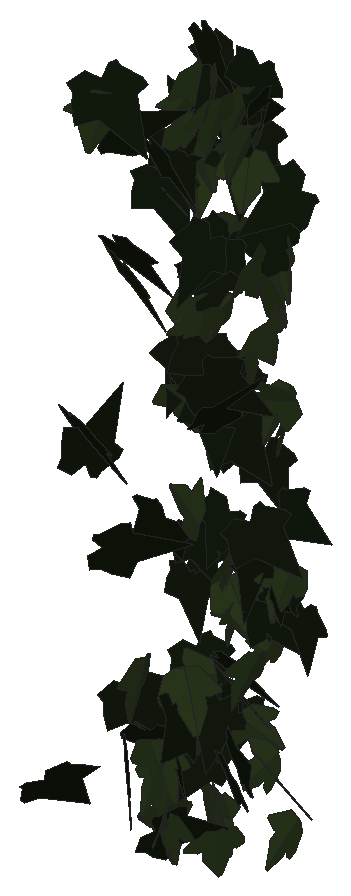
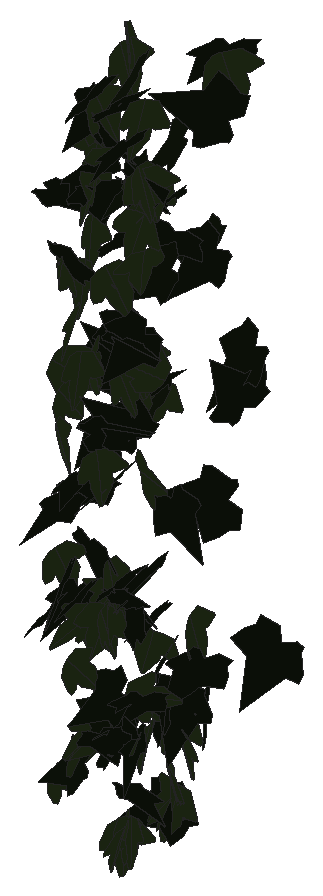
# SketchUp Ruby script. Lengths in inches.
U = 1.inch
M = Sketchup.active_model
def pt(a) = Geom::Point3d.new(a.map { |v| v * U })
def face(e, loops, mat)
  f = e.add_face(loops[0].map { |a| pt(a) })
  loops[1..].each { |l| e.add_face(l.map { |a| pt(a) }).erase! }
  f.material = f.back_material = mat if mat
  f
end
# faces: each face lists its corners as indices into pts; further lists are holes
def faces(e, pts, list, mat = nil) = list.each { |f| face(e, (f[0].is_a?(Array) ? f : [f]).map { |l| l.map { |i| pts[i] } }, mat) }
# xy, xz, yz: faces in a plane at the given z, y or x. An outline is a flat list of corners, or four numbers for a rectangle; further outlines are holes
def ring(l) = l.size == 4 ? [[l[0], l[1]], [l[2], l[1]], [l[2], l[3]], [l[0], l[3]]] : l.each_slice(2).to_a
def flat(e, list, mat, &to3) = list.each { |f| face(e, (f[0].is_a?(Array) ? f : [f]).map { |l| ring(l).map { |u, v| to3.(u, v) } }, mat) }
def xy(e, z, list, mat = nil) = flat(e, list, mat) { |x, y| [x, y, z] }
def xz(e, y, list, mat = nil) = flat(e, list, mat) { |x, z| [x, y, z] }
def yz(e, x, list, mat = nil) = flat(e, list, mat) { |y, z| [x, y, z] }
def lines(e, pts, list) = list.each { |a, b| e.add_line(pt(pts[a]), pt(pts[b])) }
# prism: a flat outline (further loops are holes) pulled along v
def prism(e, loops, v, mat = nil)
  f = face(e, loops, mat); d = Geom::Vector3d.new(v.map { |x| x * U })
  f.pushpull(f.normal.samedirection?(d) ? d.length : -d.length)
end
def box(e, o, s, mat = nil) = prism(e, [[o, [o[0] + s[0], o[1], o[2]], [o[0] + s[0], o[1] + s[1], o[2]], [o[0], o[1] + s[1], o[2]]]], [0, 0, s[2]], mat)
def at(x, y, z, deg = 0) = Geom::Transformation.translation(pt([x, y, z])) * Geom::Transformation.rotation(ORIGIN, Z_AXIS, deg.degrees)
def axes(o, x, y, z) = Geom::Transformation.new([*x, 0, *y, 0, *z, 0, *pt(o).to_a, 1])
def part(name) = M.definitions.add(name)
# library, detail: a bought-in or finely detailed component or shape, given as its bounding box
def library(name, o, s) = part(name).tap { |d| box(d.entities, o, s) }
def detail(e, o, s) = box(e.add_group.entities, o, s)
def put(e, d, t, mat = nil) = e.add_instance(d, t).tap { |i| i.material = mat if mat }
def group(e, t, mat = nil) = e.add_group.tap { |g| g.transformation = t; g.material = mat if mat }.entities
root = M.entities
M.materials.add("efeu1").color = [18, 25, 13]
M.materials.add("efeu2").color = [43, 57, 29]
c1 = part("ivyleaf_9")
p = [[1.54,2.16,1.25],[1.36,2.04,1.19],[-0.21,0.99,0.68],[-0.71,1.11,0.82],[-0.85,0.86,0.67],[-0.8,0.17,0.21],
  [-0.9,-0.01,0.1],[-0.67,-0.16,-0.02],[-0.08,-0.08,-0.05],[-0.03,-0.6,-0.4],[0.65,-0.88,-0.66],[0.83,-0.6,-0.49],
  [1.29,-0.42,-0.43],[1.8125,-0.07,-0.26],[1.21,0.44,0.15]]
faces(c1.entities,p,[[0,1,2,3,4,5,6,7,8,9,10,11,12,13,14]],"efeu1")
c2 = part("ivyleaf_10")
p = [[0,0.5,-0.03],[-0.0625,2.02,-0.43],[-0.19,2.01,-0.46],[-0.54,1.05,-0.29],[-0.52,0.625,-0.18],[-0.83,0.76,-0.28],
  [-1.16,0.64,-0.33],[-1.15,0.33,-0.24],[-0.77,-0.39,0.02],[-0.3,-0.51,0.16],[0.04,-0.48,0.23],[-0.02,2.01,-0.4375],
  [-0.06,2.01,-0.43],[0.04,-0.49,0.23],[0.67,-0.49,0.14],[1.38,0.36,-0.2],[1.375,0.51,-0.24],[0.81,0.65,-0.19],
  [0.62,0.59,-0.15],[0.6,1.09,-0.28],[0.5,1.23,-0.31]]
faces(c2.entities,p,[[0,1,2,3,4,5,6,7,8,9,10],[11,12,0,13,14,15,16,17,18,19,20]],"efeu2")
put(root,c1,axes([509.43,133.33,219.33],[-0.07106,-0.77175,0.46903],[0.10896,-0.47437,-0.76402],[0.8965,-0.00352,0.13004]))
put(root,c2,axes([510.06,132.71,207.74],[-0.8093,0.2525,0.27731],[-0.29187,0.03106,-0.82047],[-0.26852,-0.79478,0.05603]))
put(root,c1,axes([509.6,125.68,225.125],[-0.26044,-0.40713,1.01858],[0.82552,0.62963,0.46794],[-0.79417,0.788,0.15237]))
put(root,c2,axes([509.68,132.23,235],[0.34261,0.90145,-0.01403],[-0.024,-0.00589,-0.96415],[-0.90124,0.34285,0.02034]))
put(root,c1,axes([510.07,132.63,209.49],[-0.87413,-0.23226,-0.09111],[0.08835,0.03251,-0.87568],[0.25312,-0.81346,-0.00898]))
put(root,c1,axes([509.39,133.1,217.37],[-0.07665,0.02325,0.83497],[0.35529,-0.73444,0.05236],[0.79136,0.33199,0.05737]))
put(root,c1,axes([509.72,123.07,212.36],[0.6654,0.8894,0.22266],[0.13803,0.17192,-1.12521],[-0.97831,0.62918,-0.00731]))
put(root,c1,axes([509.26,131.03,234.0625],[0.93232,-0.34092,0.09087],[0.07451,-0.06071,-0.9922],[0.34487,0.93477,-0.0313]))
put(root,c2,axes([510.03,131.67,238.36],[-0.56572,-0.76176,0.26306],[-0.04096,-0.29381,-0.93889],[0.80486,-0.55038,0.13712]))
put(root,c1,axes([509.43,127.84,233.51],[1.09135,0.08087,-0.04492],[-0.04662,-0.00205,-1.05429],[-0.08735,1.01143,0.00146]))
put(root,c1,axes([510.04,132.28,212.05],[0.60792,0.03971,-0.70162],[-0.70045,0.1091,-0.60073],[0.0567,0.92192,0.10131]))
put(root,c1,axes([509.56,128.4,213.99],[-0.05655,-0.48604,-0.89596],[0.09111,0.85737,-0.50839],[1.06439,-0.09921,-0.00408]))
put(root,c1,axes([509.5,130.4,235.42],[-0.36524,-0.489,-0.76479],[0.59667,0.49718,-0.60806],[0.74408,-0.63872,0.1122]))
put(root,c2,axes([510.03,131.84,238.53],[0.0869,-0.97179,0.05974],[-0.00173,-0.06013,-0.97565],[0.97363,0.08663,-0.00707]))
put(root,c2,axes([509.9375,131.73,211.81],[-0.2319,0.86942,0.06748],[-0.10839,0.04173,-0.92693],[-0.93532,-0.2204,0.09069]))
put(root,c2,axes([510.45,131.67,213.4],[-0.11436,-0.10303,0.92284],[-0.44905,-0.80772,-0.14582],[0.81277,-0.46076,0.04928]))
put(root,c1,axes([510.33,133.125,218.96],[-0.86955,-0.17617,-0.02814],[0.03969,-0.04159,-0.85568],[0.18836,-0.80452,0.0504]))
put(root,c2,axes([510.09,129.67,207.88],[-1.06171,0.04755,-0.05074],[0.05296,0.0039,-1.02356],[-0.05108,-0.98427,-0.0065]))
put(root,c1,axes([509.62,132.41,213.9375],[0.01797,-0.70626,-0.60136],[0.21065,0.58886,-0.68529],[0.90336,-0.12327,0.17176]))
put(root,c1,axes([510.6875,130.98,237.37],[0.05271,0.33885,0.90179],[-0.69809,0.63722,-0.22114],[-0.72358,-0.59008,0.27904]))
put(root,c1,axes([509.74,131.83,217.45],[0.14195,-0.88574,-0.02827],[-0.00305,0.02814,-0.89704],[0.88618,0.14198,0.00144]))
put(root,c1,axes([510.6875,129,221.5],[0.2465,0.28682,-0.9281],[-0.88422,-0.38625,-0.34688],[-0.49296,0.83623,0.15811]))
put(root,c2,axes([510.39,129.7,207.65],[0.01164,-0.02182,1.01459],[-0.47332,0.89742,0.02473],[-0.89769,-0.47347,0.00012]))
put(root,c2,axes([510.15,131.92,236.31],[-0.9515,0.00766,-0.18123],[0.17924,-0.10887,-0.94566],[-0.02784,-0.96247,0.10552]))
put(root,c1,axes([509.93,131.95,231.05],[0.75543,0.52185,0.13154],[0.12521,0.05604,-0.90725],[-0.56624,0.70861,-0.02512]))
put(root,c2,axes([510.16,129.66,208.82],[0.74121,-0.70278,0.04986],[0.04945,-0.02228,-1.02144],[0.75916,0.68762,0.01785]))
put(root,c2,axes([509.8,131.42,228.96],[-0.2816,-0.37519,0.82169],[0.43763,0.67881,0.47432],[-0.83712,0.48108,-0.02844]))
put(root,c1,axes([509.84,124.74,227.29],[1.17306,-0.10964,-0.31105],[-0.31406,0.09259,-1.1336],[0.14045,1.12278,0.06311]))
put(root,c1,axes([509.82,130.72,236.91],[0.20947,-0.8926,-0.17498],[0.03574,0.17887,-0.94723],[0.98033,0.1842,0.07192]))
put(root,c2,axes([510.24,128.96,210.45],[0.8597,-0.59571,-0.01232],[-0.00625,0.01204,-1.03399],[0.64346,0.79601,0.00642]))
put(root,c2,axes([510.55,125.64,241.05],[-0.5616,-0.88248,0.33406],[-0.10765,-0.31323,-1.06278],[1.00852,-0.52485,0.07258]))
put(root,c1,axes([509.96,131.55,219.66],[0.36728,-0.74157,-0.37263],[-0.08365,0.37233,-0.82343],[0.8257,0.36758,0.08232]))
put(root,c1,axes([510.36,128.68,212.2],[0.83054,0.53659,-0.41955],[-0.36622,-0.21894,-0.97513],[-0.62574,0.84035,0.01384]))
put(root,c2,axes([510.28,128.0625,215.23],[0.20983,-0.98068,0.28092],[0.19545,-0.23728,-1.03132],[1.08105,0.23325,0.13194]))
put(root,c1,axes([510.21,133.48,219.61],[-0.22952,-0.81169,0.32932],[0.02334,-0.34598,-0.83649],[0.87564,-0.20353,0.10862]))
put(root,c1,axes([509.86,127.74,211.46],[-0.0249,-0.0004,-1.09458],[1.07455,-0.34331,-0.02253],[-0.37067,-0.99519,0.00821]))
put(root,c1,axes([509.76,126.68,220.91],[0.30691,0.57861,-0.88494],[0.33021,0.79541,0.66871],[1.06112,-0.41488,0.04786]))
put(root,c1,axes([510.07,129.45,207.47],[0.03422,0.43216,-0.90682],[0.07695,0.86903,0.45064],[1.0482,-0.07791,-0.00347]))
put(root,c1,axes([510.42,132.61,230.91],[-0.71795,-0.46742,-0.41007],[0.43629,0.06763,-0.84093],[0.44305,-0.82404,0.16358]))
put(root,c2,axes([510.62,132.46,229.02],[-0.01852,-0.91326,0.22885],[-0.0026,-0.22884,-0.91344],[0.94149,-0.0186,0.00198]))
put(root,c2,axes([510.41,128.92,211.3],[-1.0325,-0.04654,-0.30942],[0.32515,-0.16941,-0.97855],[-0.00712,-0.98681,0.18259]))
put(root,c2,axes([510.4,130.76,237.77],[-0.51607,-0.69102,-0.53281],[0.39573,0.36636,-0.85844],[0.77769,-0.64498,0.08324]))
put(root,c2,axes([510.07,132.96,207.2],[0.16278,-0.33966,0.83601],[0.78088,-0.37271,-0.30347],[0.45222,0.76583,0.22309]))
put(root,c2,axes([510.58,132.67,207.12],[-0.21816,0.84236,0.01689],[-0.00053,0.01659,-0.90088],[-0.90992,-0.20198,-0.00353]))
put(root,c1,axes([509.91,126.51,239.08],[0.32091,-0.01017,1.09752],[1.10805,0.25969,-0.29783],[-0.26708,1.06514,0.08309]))
put(root,c1,axes([510.58,130.75,227.85],[-0.32285,-0.85758,0.21738],[0.00785,-0.23416,-0.91216],[0.88466,-0.31089,0.08742]))
put(root,c2,axes([510.77,131.05,227.35],[0.18598,-0.8146,-0.43777],[0.11773,0.46376,-0.81294],[0.91725,0.10564,0.19311]))
put(root,c2,axes([510.9375,130.98,229.44],[-0.33356,-0.93089,0.08302],[-0.02373,-0.07969,-0.98883],[0.93428,-0.33438,0.00452]))
put(root,c1,axes([510.31,130.76,226.78],[0.44544,-0.77207,0.27374],[0.1962,-0.20197,-0.8889],[0.79532,0.48224,0.06597]))
put(root,c1,axes([510.26,132.15,226.25],[-0.01284,-0.03101,0.9233],[0.9576,-0.05476,0.01036],[0.05873,0.88618,0.03295]))
put(root,c1,axes([510.17,127.29,232.98],[0.63011,-0.72767,0.43253],[0.32063,-0.29446,-0.96895],[0.8465,0.6532,0.04505]))
put(root,c1,axes([510.74,132.4375,212.54],[-0.6482,-0.15584,-0.66212],[0.64227,0.16097,-0.66665],[0.224,-0.91249,-0.00452]))
put(root,c1,axes([510.47,125.59,241.98],[0.09469,-0.8526,-0.6817],[0.26966,0.65582,-0.85243],[1.12974,-0.08508,0.2606]))
put(root,c2,axes([511.23,131.59,206.63],[-0.54604,-0.76578,-0.05381],[0.0381,0.03892,-0.94048],[0.76672,-0.54731,0.00841]))
put(root,c2,axes([511.12,129.49,226.93],[-0.84642,-0.34341,-0.21699],[0.20364,0.07523,-0.9134],[0.35149,-0.87054,0.00667]))
put(root,c1,axes([510.83,131.1,238.03],[0.83199,-0.46646,-0.20758],[-0.17598,0.11057,-0.95378],[0.47928,0.85034,0.01014]))
put(root,c1,axes([511.9375,132.75,225.93],[-0.50923,-0.44858,-0.64625],[-0.41032,-0.50536,0.67411],[-0.67119,0.64928,0.0782]))
put(root,c2,axes([511.23,130.31,240.6],[-0.31499,-0.91313,-0.34822],[0.22971,0.28643,-0.9589],[0.9499,-0.37207,0.11642]))
put(root,c2,axes([511.6,132.06,233.33],[-0.52405,-0.70315,0.39512],[-0.23706,-0.31611,-0.87695],[0.77094,-0.57517,-0.00108]))
put(root,c1,axes([511.29,133.07,211.88],[-0.57033,-0.65308,-0.18702],[0.11964,0.14381,-0.86704],[0.66871,-0.58272,-0.00438]))
put(root,c1,axes([510.79,132.51,213.78],[0.92273,-0.10296,0.15482],[0.15528,-0.00435,-0.92837],[0.10226,0.93562,0.01272]))
put(root,c2,axes([511.5625,132.91,224.83],[-0.36769,-0.85905,0.01417],[-0.00385,-0.01377,-0.93443],[0.85916,-0.3677,0.00188]))
put(root,c1,axes([510.96,129.38,210.76],[0.00483,-0.12634,1.01915],[0.27407,-0.98204,-0.12303],[0.9897,0.27256,0.0291]))
put(root,c1,axes([511.03,131.76,239.82],[0.3607,-0.78077,-0.48096],[-0.0305,0.50633,-0.84482],[0.91651,0.32413,0.16117]))
put(root,c1,axes([511.21,130.97,228.31],[-0.2122,-0.8904,-0.37501],[0.13351,0.35324,-0.91426],[0.95688,-0.24674,0.0444]))
put(root,c1,axes([511.34,131.49,212.58],[-0.28978,-0.89135,-0.05788],[0.00994,0.05763,-0.93723],[0.89317,-0.28983,-0.00835]))
put(root,c1,axes([511.1,132.07,223.93],[0.62187,-0.53026,-0.4216],[-0.09413,0.49911,-0.7666],[0.67087,0.56157,0.28324]))
put(root,c2,axes([512.24,128.96,222.14],[0.25756,0.06853,1.0147],[-0.99501,0.23356,0.23679],[-0.21043,-1.02049,0.12234]))
put(root,c1,axes([511.17,127.82,238.3125],[0.85378,-0.54645,-0.14226],[-0.10144,0.10527,-1.01312],[0.55548,0.85913,0.03365]))
put(root,c2,axes([511.8125,131.71,218.97],[0.17029,-0.88741,-0.064],[-0.00834,0.06357,-0.9036],[0.88968,0.17045,0.00378]))
put(root,c2,axes([511.8,132.14,216.8],[0.22701,-0.85457,0.14964],[0.05833,-0.1393,-0.88397],[0.86561,0.23351,0.02032]))
put(root,c1,axes([511.14,132.7,212.68],[0.45169,-0.54252,0.60462],[0.44265,-0.41569,-0.70368],[0.68114,0.62991,0.05636]))
put(root,c1,axes([511.59,129.11,212.92],[-0.03881,-0.66205,0.79895],[-0.04569,-0.79764,-0.66319],[1.0366,-0.05994,0.00068]))
put(root,c2,axes([511.99,131.97,216.85],[-0.88785,-0.31401,-0.19448],[0.17682,0.08319,-0.94155],[0.32429,-0.90509,-0.01906]))
put(root,c1,axes([511.57,130.34,242.33],[0.68017,-0.70973,-0.16453],[-0.12883,0.10438,-0.98281],[0.71707,0.69195,-0.0205]))
put(root,c2,axes([511.65,129.11,214.68],[0.91924,0.33945,0.34972],[0.32844,0.12013,-0.97991],[-0.36008,0.97615,-0.00102]))
put(root,c1,axes([512.04,131.41,241],[-0.45415,-0.78601,0.39722],[-0.02701,-0.43428,-0.89024],[0.88027,-0.41885,0.17762]))
put(root,c1,axes([512.05,130.53,226.4375],[-0.15953,-0.94984,-0.18853],[0.02592,0.18681,-0.96313],[0.96802,-0.16154,-0.00528]))
put(root,c2,axes([511.99,132.4,211.65],[-0.54868,-0.4166,-0.6461],[0.56042,0.3266,-0.68652],[0.52624,-0.78219,0.05746]))
put(root,c2,axes([511.91,131.57,217.77],[0.76922,0.24532,0.51473],[0.47896,0.19104,-0.80681],[-0.30941,0.90563,0.03076]))
put(root,c2,axes([512.49,133.33,214.89],[-0.09013,-0.66178,0.58659],[0.02177,-0.59111,-0.66353],[0.88406,-0.05292,0.07614]))
put(root,c1,axes([512.54,131.83,237.11],[-0.46453,-0.82134,-0.2699],[0.10923,0.24819,-0.94325],[0.85763,-0.47649,-0.02606]))
put(root,c2,axes([512.82,132.5,228.92],[-0.18966,-0.88656,-0.28977],[0.11547,0.27111,-0.90504],[0.92554,-0.21549,0.05353]))
put(root,c1,axes([512.3125,131.09,209.91],[0.10125,-0.4855,0.82162],[0.29584,-0.76957,-0.4912],[0.90733,0.3051,0.06847]))
put(root,c1,axes([512.81,130.18,233.88],[-0.36419,-0.79718,0.42304],[-0.10122,-0.41723,-0.87337],[0.89678,-0.37084,0.07323]))
put(root,c2,axes([512.9,131.6875,237.93],[0.05026,-0.80906,0.56172],[0.08325,-0.55694,-0.80964],[0.98141,0.08868,0.03991]))
put(root,c2,axes([512.82,132.77,210.05],[-0.30246,-0.13498,0.86565],[0.27892,-0.88297,-0.04022],[0.83053,0.24738,0.32876]))
put(root,c2,axes([513.01,131.61,237.21],[-0.74841,0.61876,0.11802],[-0.08822,0.07851,-0.97107],[-0.62371,-0.75358,-0.00426]))
put(root,c1,axes([512.72,130.64,225.47],[0.03759,-0.57969,-0.79119],[-0.02092,0.79112,-0.58063],[0.9806,0.0391,0.01794]))
put(root,c1,axes([512.73,133,217.84],[0.06709,-0.87143,0.19437],[0.00813,-0.19432,-0.87398],[0.89281,0.06725,-0.00665]))
put(root,c2,axes([512.95,132.14,216.47],[0.08727,0.41807,0.81576],[0.07481,0.81346,-0.4249],[-0.91359,0.10655,0.04313]))
put(root,c1,axes([513.89,130.18,238.86],[-0.54688,0.44439,0.689],[-0.51688,0.45602,-0.70439],[-0.63643,-0.75222,-0.01998]))
put(root,c1,axes([512.75,131.72,238.01],[0.08293,-0.86405,-0.46532],[0.09364,0.47181,-0.85942],[0.9769,0.02812,0.12188]))
put(root,c1,axes([513.05,131.54,219.8125],[-0.75377,-0.12484,-0.60898],[0.59361,0.13963,-0.76337],[0.18457,-0.95892,-0.03188]))
put(root,c1,axes([512.83,132.5,223.62],[0.15795,-0.83646,-0.36525],[-0.01635,0.36803,-0.84989],[0.91259,0.15137,0.04799]))
put(root,c1,axes([512.71,130.97,210.57],[-0.03432,-0.10138,0.94975],[0.39345,-0.86749,-0.07838],[0.87035,0.38816,0.07289]))
put(root,c1,axes([512.65,132.65,209.85],[0.79752,-0.46356,0.2332],[0.20411,-0.11288,-0.92244],[0.47708,0.82321,0.00483]))
put(root,c2,axes([513.38,132.26,230.95],[-0.44061,0.77275,0.36419],[-0.18293,0.31492,-0.88954],[-0.83446,-0.47706,0.00271]))
put(root,c1,axes([514.12,132,233.18],[-0.60291,0.29819,0.70138],[-0.63986,0.2878,-0.67239],[-0.41404,-0.87898,0.01778]))
put(root,c2,axes([513.5,130.32,240.23],[0.00009,-0.97415,0.37068],[0.0403,-0.3704,-0.97342],[1.04151,0.01442,0.03763]))
put(root,c1,axes([513.63,128.01,235.09],[-0.88772,-0.23885,-0.3304],[0.329,0.04785,-0.91855],[0.24077,-0.946,0.03696]))
put(root,c2,axes([513.6,132.89,225.47],[0.45881,-0.81451,0.04054],[0.02675,-0.03146,-0.93481],[0.81508,0.45952,0.00785]))
put(root,c1,axes([513.35,131.4,241.04],[0.02124,-0.98035,0.17877],[-0.03235,-0.17939,-0.97993],[0.99599,0.01508,-0.03564]))
put(root,c1,axes([513.17,128.58,226.77],[0.40373,0.96973,-0.07118],[0.01788,0.06966,1.05037],[0.97218,-0.404,0.01024]))
put(root,c1,axes([513.14,128.51,228.78],[0.04984,-0.09772,-1.04658],[0.35721,0.98697,-0.07514],[0.98857,-0.35171,0.07992]))
put(root,c2,axes([513.32,131.09,227.875],[0.16912,-0.27585,0.91667],[0.58728,-0.70521,-0.32056],[0.75596,0.60956,0.04397]))
put(root,c1,axes([513.78,132.0625,218.52],[0.44296,-0.25191,-0.78186],[-0.62415,0.47428,-0.50643],[0.53404,0.76326,0.05663]))
put(root,c2,axes([513.85,130.47,215.69],[-0.00244,-0.90618,0.38921],[0.01294,-0.3892,-0.90609],[0.98614,0.00286,0.01286]))
put(root,c2,axes([514.04,130.91,232.25],[-0.88842,0.3289,0.27472],[-0.25422,0.10455,-0.94729],[-0.34499,-0.92402,-0.0094]))
put(root,c1,axes([513.61,131.79,217.55],[0.12539,-0.56618,-0.78224],[-0.14278,0.76926,-0.57968],[0.95502,0.18935,0.01604]))
put(root,c1,axes([514.13,129.88,239.8],[-0.13897,0.20363,-0.96166],[-0.57139,0.77356,0.24637],[0.79986,0.58798,0.00891]))
put(root,c2,axes([514.11,127.68,242.15],[0.48111,-0.84518,-0.38706],[-0.11407,0.37886,-0.96906],[0.92257,0.4876,0.08203]))
put(root,c2,axes([514.19,129.66,239.17],[-0.03925,-0.99115,0.30908],[-0.02989,-0.30809,-0.99178],[1.03779,-0.04635,-0.01687]))
put(root,c2,axes([514.22,127.83,241.18],[-0.12496,-1.02613,0.13782],[0.02584,-0.14187,-1.03284],[1.03503,-0.12035,0.04243]))
put(root,c2,axes([514.06,132.02,226.71],[-0.09984,-0.7118,0.60771],[0.20724,-0.6128,-0.68372],[0.9127,0.06128,0.22173]))
put(root,c2,axes([514.32,132.06,218.92],[-0.37942,-0.75499,0.40283],[0.06302,-0.46411,-0.81048],[0.85341,-0.30139,0.23894]))
put(root,c2,axes([514.12,129.76,237.95],[0.93385,0.33849,0.00534],[0.00426,0.00391,-0.9933],[-0.3385,0.93386,0.00222]))
put(root,c1,axes([514.02,132,221.76],[0.29119,-0.31754,-0.82236],[-0.18812,0.82372,-0.38468],[0.86123,0.2873,0.19402]))
put(root,c2,axes([515.07,130.83,227.34],[0.23145,0.36401,-0.91335],[-0.9823,0.12612,-0.19866],[0.04245,0.93374,0.3829]))
put(root,c2,axes([514.47,129.62,233.61],[0.09735,-0.93087,-0.39747],[0.02899,0.40171,-0.93369],[1.01176,0.07806,0.065]))
put(root,c1,axes([513.94,130.33,221.83],[0.15617,-0.55902,-0.7958],[0.18659,0.80824,-0.53115],[0.95445,-0.06654,0.23405]))
put(root,c2,axes([514.01,132.11,232.96],[0.70979,-0.33728,0.56936],[0.54186,-0.18308,-0.78396],[0.37988,0.89132,0.05442]))
put(root,c1,axes([514.12,133.22,216.79],[0.13762,-0.86894,0.15465],[0.02863,-0.15204,-0.87976],[0.88213,0.1405,0.00443]))
put(root,c1,axes([515.05,131.69,236.11],[-0.87092,-0.3691,0.27433],[-0.25902,-0.09177,-0.94578],[0.38001,-0.90849,-0.01592]))
put(root,c2,axes([514.62,131.8,208.12],[-0.12905,-0.44674,0.81263],[0.2704,-0.80293,-0.39847],[0.88703,0.17977,0.23969]))
